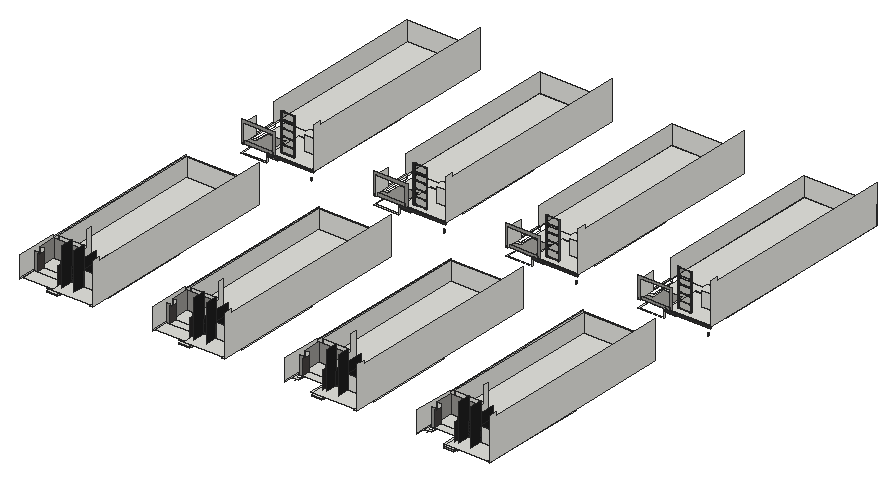
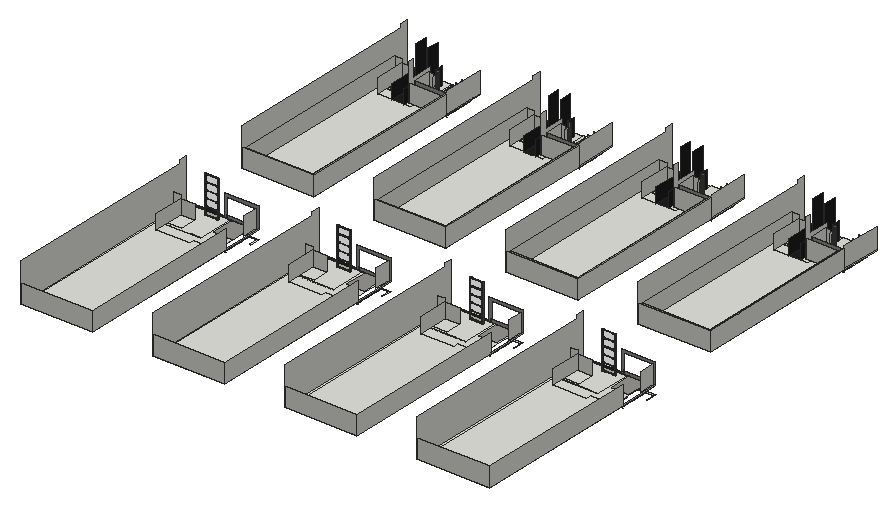
# SketchUp Ruby script. Lengths in inches.
U = 1.inch
M = Sketchup.active_model
def pt(a) = Geom::Point3d.new(a.map { |v| v * U })
def face(e, loops, mat)
  f = e.add_face(loops[0].map { |a| pt(a) })
  loops[1..].each { |l| e.add_face(l.map { |a| pt(a) }).erase! }
  f.material = f.back_material = mat if mat
  f
end
# faces: each face lists its corners as indices into pts; further lists are holes
def faces(e, pts, list, mat = nil) = list.each { |f| face(e, (f[0].is_a?(Array) ? f : [f]).map { |l| l.map { |i| pts[i] } }, mat) }
# xy, xz, yz: faces in a plane at the given z, y or x. An outline is a flat list of corners, or four numbers for a rectangle; further outlines are holes
def ring(l) = l.size == 4 ? [[l[0], l[1]], [l[2], l[1]], [l[2], l[3]], [l[0], l[3]]] : l.each_slice(2).to_a
def flat(e, list, mat, &to3) = list.each { |f| face(e, (f[0].is_a?(Array) ? f : [f]).map { |l| ring(l).map { |u, v| to3.(u, v) } }, mat) }
def xy(e, z, list, mat = nil) = flat(e, list, mat) { |x, y| [x, y, z] }
def xz(e, y, list, mat = nil) = flat(e, list, mat) { |x, z| [x, y, z] }
def yz(e, x, list, mat = nil) = flat(e, list, mat) { |y, z| [x, y, z] }
def lines(e, pts, list) = list.each { |a, b| e.add_line(pt(pts[a]), pt(pts[b])) }
# prism: a flat outline (further loops are holes) pulled along v
def prism(e, loops, v, mat = nil)
  f = face(e, loops, mat); d = Geom::Vector3d.new(v.map { |x| x * U })
  f.pushpull(f.normal.samedirection?(d) ? d.length : -d.length)
end
def box(e, o, s, mat = nil) = prism(e, [[o, [o[0] + s[0], o[1], o[2]], [o[0] + s[0], o[1] + s[1], o[2]], [o[0], o[1] + s[1], o[2]]]], [0, 0, s[2]], mat)
def at(x, y, z, deg = 0) = Geom::Transformation.translation(pt([x, y, z])) * Geom::Transformation.rotation(ORIGIN, Z_AXIS, deg.degrees)
def axes(o, x, y, z) = Geom::Transformation.new([*x, 0, *y, 0, *z, 0, *pt(o).to_a, 1])
def part(name) = M.definitions.add(name)
# library, detail: a bought-in or finely detailed component or shape, given as its bounding box
def library(name, o, s) = part(name).tap { |d| box(d.entities, o, s) }
def detail(e, o, s) = box(e.add_group.entities, o, s)
def put(e, d, t, mat = nil) = e.add_instance(d, t).tap { |i| i.material = mat if mat }
def group(e, t, mat = nil) = e.add_group.tap { |g| g.transformation = t; g.material = mat if mat }.entities
root = M.entities
M.materials.add("Aluminum_Polished").color = [83, 85, 85]
M.materials.add("Glass_Window_Neutral").color = [0, 0, 0]
M.materials["Glass_Window_Neutral"].alpha = 0.125
M.materials.add("[Color M07]").color = [58, 58, 58]
M.materials.add("[Color M08]").color = [30, 30, 30]
M.materials.add("[Field Square Tile]").color = [211, 167, 108]
M.materials.add("[Granite Dark Gray]").color = [38, 37, 37]
M.materials.add("[Granite Light Gray]").color = [149, 148, 144]
M.materials.add("[Granite Tile]1").color = [68, 65, 63]
c1 = part("Group\#7")
xy(c1.entities,0,[[6,0,4.45,0.2,3,0.8,1.76,1.76,0.8,3,0.2,4.45,0,6,0.2,7.55,0.8,9,1.76,10.24,3,11.2,4.45,11.8,6,12,7.55,11.8,9,11.2,10.24,10.24,11.2,9,11.8,7.55,12,6,11.8,4.45,11.2,3,10.24,1.76,9,0.8,7.55,0.2]])
xy(c1.entities,37,[[6,0,7.55,0.2,9,0.8,10.24,1.76,11.2,3,11.8,4.45,12,6,11.8,7.55,11.2,9,10.24,10.24,9,11.2,7.55,11.8,6,12,4.45,11.8,3,11.2,1.76,10.24,0.8,9,0.2,7.55,0,6,0.2,4.45,0.8,3,1.76,1.76,3,0.8,4.45,0.2]],"[Granite Tile]1")
p = [[4.45,0.2,0],[6,0,0],[6,0,37],[4.45,0.2,37],[7.55,0.2,0],[7.55,0.2,37],
  [3,0.8,0],[3,0.8,37],[9,0.8,0],[9,0.8,37],[1.76,1.76,0],[1.76,1.76,37],
  [10.24,1.76,0],[10.24,1.76,37],[0.8,3,0],[0.8,3,37],[11.2,3,0],[11.2,3,37],
  [0.2,4.45,0],[0.2,4.45,37],[11.8,4.45,0],[11.8,4.45,37],[0,6,0],[0,6,37],
  [12,6,0],[12,6,37],[0.2,7.55,0],[0.2,7.55,37],[11.8,7.55,0],[11.8,7.55,37],
  [0.8,9,0],[0.8,9,37],[11.2,9,0],[11.2,9,37],[1.76,10.24,0],[1.76,10.24,37],
  [10.24,10.24,0],[10.24,10.24,37],[3,11.2,0],[3,11.2,37],[9,11.2,0],[9,11.2,37],
  [4.45,11.8,0],[4.45,11.8,37],[7.55,11.8,0],[7.55,11.8,37],[6,12,0],[6,12,37]]
faces(c1.entities,p,[[0,1,2,3],[1,4,5,2],[6,0,3,7],[4,8,9,5],[10,6,7,11],[8,12,13,9],[14,10,11,15],[12,16,17,13],
  [18,14,15,19],[16,20,21,17],[22,18,19,23],[20,24,25,21],[26,22,23,27],[24,28,29,25],[30,26,27,31],[28,32,33,29],
  [34,30,31,35],[32,36,37,33],[38,34,35,39],[36,40,41,37],[42,38,39,43],[40,44,45,41],[46,42,43,47],[44,46,47,45]],"[Granite Tile]1")
c2 = part("Group\#54")
box(c2.entities,[0,0,0],[2,1,28])
c3 = part("Group\#56")
p = [[0.11,0.32,0.14],[0.11,0.69,0.14]]
lines(c3.entities,p,[[0,1]])
g1 = group(c3.entities,at(0.11,0,0))
prism(g1,[[[0,0.24,0],[0,0.32,0.14],[0,0.24,0.27],[0,0.08,0.27],[0,0,0.14],[0,0.08,0]]],[-0.11,0,0])
c4 = part("Ver Glass Railing")
g2 = group(c4.entities,at(0,0,0),"Aluminum_Polished")
box(g2,[0,0,0],[2,185,2])
g3 = group(c4.entities,at(0,0,2),"Aluminum_Polished")
p = [[1.41,1,0],[1.41,36.8,0],[1.41,184,0],[1.29,184,0],[1.29,1,0],[1.29,36.8,0],
  [1.41,184,28],[1.29,184,28],[1.41,148.2,28],[1.29,148.2,28],[1.41,1,28],[1.29,1,28],
  [1.29,111.4,28],[1.29,111.4,0],[1.41,111.4,0],[1.41,111.4,28],[1.29,110.4,0],[1.29,110.4,28],
  [1.41,110.4,28],[1.41,110.4,0],[1.29,74.6,28],[1.29,74.6,0],[1.41,74.6,0],[1.41,74.6,28],
  [1.29,73.6,0],[1.29,73.6,28],[1.41,73.6,28],[1.41,73.6,0],[1.29,148.2,0],[1.41,148.2,0],
  [1.29,147.2,0],[1.29,147.2,28],[1.41,147.2,28],[1.41,147.2,0],[1.29,37.8,28],[1.29,37.8,0],
  [1.41,37.8,0],[1.41,37.8,28],[1.29,36.8,28],[1.41,36.8,28]]
lines(g3,p,[[0,1],[2,3],[4,5],[6,7],[6,8],[7,9],[10,11],[2,6],[3,7],[0,4],[11,4],[10,0],
  [12,13],[14,15],[16,17],[18,19],[20,21],[22,23],[24,25],[26,27],[27,22],[24,21],[23,26],[20,25],
  [9,28],[29,8],[30,31],[32,33],[33,29],[30,28],[8,32],[9,31],[34,35],[36,37],[5,38],[39,1],
  [1,36],[5,35],[37,39],[14,33],[19,14],[22,19],[36,27],[13,30],[16,13],[21,16],[35,24],[15,18],
  [12,17],[29,2],[28,3],[18,23],[32,15],[17,20],[31,12],[26,37],[25,34],[34,38],[39,10],[38,11]])
g4 = group(g3,at(1.79,1,0))
box(g4,[-0.5,0,0],[0.125,183,28],"Glass_Window_Neutral")
g5 = group(g3,at(0,184,28))
box(g5,[0,-184,0],[2.5,185,1])
put(g3,c2,axes([2,185,28],[-1,0,0],[0,-1,0],[0,0,-1]))
put(g3,c2,axes([2,1,28],[-1,0,0],[0,-1,0],[0,0,-1]))
put(g3,c2,axes([2,111.4,28],[-1,0,0],[0,-1,0],[0,0,-1]))
put(g3,c2,axes([2,74.6,28],[-1,0,0],[0,-1,0],[0,0,-1]))
g6 = group(g3,at(2,148.2,28))
box(g6,[-2,-1,-28],[2,1,28])
put(g3,c2,axes([2,37.8,28],[-1,0,0],[0,-1,0],[0,0,-1]))
put(g3,c3,at(1.17,146.31,24.26))
put(g3,c3,axes([1.17,148.89,24.54],[1,0,0],[0,-1,0],[0,0,-1]))
put(g3,c3,axes([1.17,148.89,4.79],[1,0,0],[0,-1,0],[0,0,-1]))
put(g3,c3,at(1.17,146.31,4.51))
put(g3,c3,at(1.17,109.51,4.51))
put(g3,c3,axes([1.17,112.09,4.79],[1,0,0],[0,-1,0],[0,0,-1]))
put(g3,c3,axes([1.17,112.09,24.54],[1,0,0],[0,-1,0],[0,0,-1]))
put(g3,c3,at(1.17,109.51,24.26))
put(g3,c3,axes([1.17,75.29,24.54],[1,0,0],[0,-1,0],[0,0,-1]))
put(g3,c3,at(1.17,72.71,4.51))
put(g3,c3,axes([1.17,75.29,4.79],[1,0,0],[0,-1,0],[0,0,-1]))
put(g3,c3,at(1.17,72.71,24.26))
put(g3,c3,axes([1.17,38.49,24.54],[1,0,0],[0,-1,0],[0,0,-1]))
put(g3,c3,at(1.17,35.91,4.51))
put(g3,c3,axes([1.17,38.49,4.79],[1,0,0],[0,-1,0],[0,0,-1]))
put(g3,c3,at(1.17,35.91,24.26))
xy(root,72.4375,[[218.97,2293.1875,388.78,2293.1875,388.78,2300.94,225.79,2300.94,225.79,2358.81,218.97,2358.81],[1097.72,2293.1875,1267.53,2293.1875,1267.53,2300.94,1104.54,2300.94,1104.54,2358.81,1097.72,2358.81],[1976.47,2293.1875,2146.28,2293.1875,2146.28,2300.94,1983.29,2300.94,1983.29,2358.81,1976.47,2358.81],[2855.22,2293.1875,3025.03,2293.1875,3025.03,2300.94,2862.04,2300.94,2862.04,2358.81,2855.22,2358.81]])
xy(root,96.1875,[[402.97,706.62,460.85,1288.43],[1281.72,706.62,1339.6,1288.43],[2160.47,706.62,2218.35,1288.43],[3039.22,706.62,3097.1,1288.43],[402.97,2542.24,460.85,3124.06],
  [1281.72,2542.24,1339.6,3124.06],[2160.47,2542.24,2218.35,3124.06],[3039.22,2542.24,3097.1,3124.06]])
xy(root,96.29,[[488.9,633.06,669.8,1213.68],[1367.65,633.06,1548.55,1213.68],[2246.4,633.06,2427.3,1213.68],[3125.15,633.06,3306.05,1213.68],[488.9,2468.68,669.8,3049.31],
  [1367.65,2468.68,1548.55,3049.31],[2246.4,2468.68,2427.3,3049.31],[3125.15,2468.68,3306.05,3049.31]])
xy(root,107.07,[[279.88,619.06,385.01,1006.15],[1158.63,619.06,1263.76,1006.15],[2037.38,619.06,2142.51,1006.15],[2916.13,619.06,3021.26,1006.15],[279.88,2454.68,385.01,2841.77],
  [1158.63,2454.68,1263.76,2841.77],[2037.38,2454.68,2142.51,2841.77],[2916.13,2454.68,3021.26,2841.77]])
xy(root,110.32,[[395.95,458.5,463.7,706.62],[1274.7,458.5,1342.45,706.62],[2153.45,458.5,2221.2,706.62],[3032.2,458.5,3099.95,706.62],[395.95,2294.125,463.7,2542.24],
  [1274.7,2294.125,1342.45,2542.24],[2153.45,2294.125,2221.2,2542.24],[3032.2,2294.125,3099.95,2542.24]],"[Granite Light Gray]")
xy(root,116.94,[[481.29,561.06,678.9,571.64],[1360.04,561.06,1557.65,571.64],[2238.79,561.06,2436.4,571.64],[3117.54,561.06,3315.15,571.64],[481.29,2396.68,678.9,2407.27],
  [1360.04,2396.68,1557.65,2407.27],[2238.79,2396.68,2436.4,2407.27],[3117.54,2396.68,3315.15,2407.27]],"[Field Square Tile]")
xy(root,118.38,[[395.95,458.5,463.7,706.62],[1274.7,458.5,1342.45,706.62],[2153.45,458.5,2221.2,706.62],[3032.2,458.5,3099.95,706.62],[463.7,465.32,481.29,465.32,481.29,633.06,475.35,633.06,475.35,706.62,463.7,706.62],
  [1342.45,465.32,1360.04,465.32,1360.04,633.06,1354.1,633.06,1354.1,706.62,1342.45,706.62],[2221.2,465.32,2238.79,465.32,2238.79,633.06,2232.85,633.06,2232.85,706.62,2221.2,706.62],[3099.95,465.32,3117.54,465.32,3117.54,633.06,3111.6,633.06,3111.6,706.62,3099.95,706.62],[475.35,633.06,640.4,706.62],[640.4,633.06,678.9,706.62],
  [1354.1,633.06,1519.15,706.62],[1519.15,633.06,1557.65,706.62],[2232.85,633.06,2397.9,706.62],[2397.9,633.06,2436.4,706.62],[3111.6,633.06,3276.65,706.62],
  [3276.65,633.06,3315.15,706.62],[395.95,2294.125,463.7,2542.24],[463.7,2294.125,481.29,2300.94],[1274.7,2294.125,1342.45,2542.24],[1342.45,2294.125,1360.04,2300.94],
  [2153.45,2294.125,2221.2,2542.24],[2221.2,2294.125,2238.79,2300.94],[3032.2,2294.125,3099.95,2542.24],[3099.95,2294.125,3117.54,2300.94],[463.7,2300.94,481.29,2300.94,481.29,2468.68,475.35,2468.68,475.35,2542.24,463.7,2542.24],
  [1342.45,2300.94,1360.04,2300.94,1360.04,2468.68,1354.1,2468.68,1354.1,2542.24,1342.45,2542.24],[2221.2,2300.94,2238.79,2300.94,2238.79,2468.68,2232.85,2468.68,2232.85,2542.24,2221.2,2542.24],[3099.95,2300.94,3117.54,2300.94,3117.54,2468.68,3111.6,2468.68,3111.6,2542.24,3099.95,2542.24],[475.35,2468.68,640.4,2542.24],[640.4,2468.68,678.9,2542.24],
  [1354.1,2468.68,1519.15,2542.24],[1519.15,2468.68,1557.65,2542.24],[2232.85,2468.68,2397.9,2542.24],[2397.9,2468.68,2436.4,2542.24],[3111.6,2468.68,3276.65,2542.24],
  [3276.65,2468.68,3315.15,2542.24]])
xy(root,118.38,[[481.29,571.64,678.9,633.06],[1360.04,571.64,1557.65,633.06],[2238.79,571.64,2436.4,633.06],[3117.54,571.64,3315.15,633.06],[481.29,2294.125,678.9,2396.68],
  [1360.04,2294.125,1557.65,2396.68],[2238.79,2294.125,2436.4,2396.68],[3117.54,2294.125,3315.15,2396.68],[481.29,2407.27,678.9,2468.68],[1360.04,2407.27,1557.65,2468.68],
  [2238.79,2407.27,2436.4,2468.68],[3117.54,2407.27,3315.15,2468.68]],"[Granite Light Gray]")
xy(root,128.5,[[[678.9,458.5,698.16,458.5,698.16,1835.625,218.97,1835.625,218.97,523.18,262.66,523.18,262.66,619.06,388.78,619.06,388.78,463.25,399.95,463.25,399.95,706.62,678.9,706.62],[225.79,539.02,225.79,1828.81,678.9,1828.81,678.9,986.46,261.53,986.46,261.53,539.02]],[[1557.65,458.5,1576.91,458.5,1576.91,1835.625,1097.72,1835.625,1097.72,523.18,1141.41,523.18,1141.41,619.06,1267.53,619.06,1267.53,463.25,1278.7,463.25,1278.7,706.62,1557.65,706.62],[1104.54,539.02,1104.54,1828.81,1557.65,1828.81,1557.65,986.46,1140.28,986.46,1140.28,539.02]],[[2436.4,458.5,2455.66,458.5,2455.66,1835.625,1976.47,1835.625,1976.47,523.18,2020.16,523.18,2020.16,619.06,2146.28,619.06,2146.28,463.25,2157.45,463.25,2157.45,706.62,2436.4,706.62],[1983.29,539.02,1983.29,1828.81,2436.4,1828.81,2436.4,986.46,2019.03,986.46,2019.03,539.02]],[[3315.15,458.5,3334.41,458.5,3334.41,1835.625,2855.22,1835.625,2855.22,523.18,2898.91,523.18,2898.91,619.06,3025.03,619.06,3025.03,463.25,3036.2,463.25,3036.2,706.62,3315.15,706.62],[2862.04,539.02,2862.04,1828.81,3315.15,1828.81,3315.15,986.46,2897.78,986.46,2897.78,539.02]],[399.95,465.32,678.9,706.62],
  [1278.7,465.32,1557.65,706.62],[2157.45,465.32,2436.4,706.62],[3036.2,465.32,3315.15,706.62],[261.53,986.46,678.9,1006.15],[1140.28,986.46,1557.65,1006.15],
  [2019.03,986.46,2436.4,1006.15],[2897.78,986.46,3315.15,1006.15],[261.53,1006.15,678.9,1010.9],[1140.28,1006.15,1557.65,1010.9],[2019.03,1006.15,2436.4,1010.9],
  [2897.78,1006.15,3315.15,1010.9],[218.97,2294.125,225.79,2358.81],[[678.9,2294.125,698.16,2294.125,698.16,3671.25,218.97,3671.25,218.97,2358.81,262.66,2358.81,262.66,2454.68,388.78,2454.68,388.78,2298.875,399.95,2298.875,399.95,2542.24,678.9,2542.24],[225.79,2374.65,225.79,3664.43,678.9,3664.43,678.9,2822.08,261.53,2822.08,261.53,2374.65]],[388.78,2294.125,399.95,2298.875],[399.95,2294.125,427.1,2298.875],
  [427.1,2294.125,427.1,2298.875,399.95,2298.875,399.95,2300.94,678.9,2300.94,678.9,2294.125],[1097.72,2294.125,1104.54,2358.81],[[1557.65,2294.125,1576.91,2294.125,1576.91,3671.25,1097.72,3671.25,1097.72,2358.81,1141.41,2358.81,1141.41,2454.68,1267.53,2454.68,1267.53,2298.875,1278.7,2298.875,1278.7,2542.24,1557.65,2542.24],[1104.54,2374.65,1104.54,3664.43,1557.65,3664.43,1557.65,2822.08,1140.28,2822.08,1140.28,2374.65]],[1267.53,2294.125,1278.7,2298.875],[1278.7,2294.125,1305.85,2298.875],
  [1305.85,2294.125,1305.85,2298.875,1278.7,2298.875,1278.7,2300.94,1557.65,2300.94,1557.65,2294.125],[1976.47,2294.125,1983.29,2358.81],[[2436.4,2294.125,2455.66,2294.125,2455.66,3671.25,1976.47,3671.25,1976.47,2358.81,2020.16,2358.81,2020.16,2454.68,2146.28,2454.68,2146.28,2298.875,2157.45,2298.875,2157.45,2542.24,2436.4,2542.24],[1983.29,2374.65,1983.29,3664.43,2436.4,3664.43,2436.4,2822.08,2019.03,2822.08,2019.03,2374.65]],[2146.28,2294.125,2157.45,2298.875],[2157.45,2294.125,2184.6,2298.875],
  [2184.6,2294.125,2184.6,2298.875,2157.45,2298.875,2157.45,2300.94,2436.4,2300.94,2436.4,2294.125],[2855.22,2294.125,2862.04,2358.81],[[3315.15,2294.125,3334.41,2294.125,3334.41,3671.25,2855.22,3671.25,2855.22,2358.81,2898.91,2358.81,2898.91,2454.68,3025.03,2454.68,3025.03,2298.875,3036.2,2298.875,3036.2,2542.24,3315.15,2542.24],[2862.04,2374.65,2862.04,3664.43,3315.15,3664.43,3315.15,2822.08,2897.78,2822.08,2897.78,2374.65]],[3025.03,2294.125,3036.2,2298.875],[3036.2,2294.125,3063.35,2298.875],
  [3063.35,2294.125,3063.35,2298.875,3036.2,2298.875,3036.2,2300.94,3315.15,2300.94,3315.15,2294.125],[399.95,2300.94,678.9,2542.24],[1278.7,2300.94,1557.65,2542.24],[2157.45,2300.94,2436.4,2542.24],[3036.2,2300.94,3315.15,2542.24],
  [261.53,2822.08,678.9,2841.77],[1140.28,2822.08,1557.65,2841.77],[2019.03,2822.08,2436.4,2841.77],[2897.78,2822.08,3315.15,2841.77],[261.53,2841.77,678.9,2846.52],
  [1140.28,2841.77,1557.65,2846.52],[2019.03,2841.77,2436.4,2846.52],[2897.78,2841.77,3315.15,2846.52]])
xy(root,128.5,[[228.78,2294.125,228.78,2358.81,262.66,2358.81,262.66,2454.68,388.78,2454.68,388.78,2298.875,232.96,2298.875,232.96,2294.125],[1107.53,2294.125,1107.53,2358.81,1141.41,2358.81,1141.41,2454.68,1267.53,2454.68,1267.53,2298.875,1111.71,2298.875,1111.71,2294.125],[1986.28,2294.125,1986.28,2358.81,2020.16,2358.81,2020.16,2454.68,2146.28,2454.68,2146.28,2298.875,1990.46,2298.875,1990.46,2294.125],[2865.03,2294.125,2865.03,2358.81,2898.91,2358.81,2898.91,2454.68,3025.03,2454.68,3025.03,2298.875,2869.21,2298.875,2869.21,2294.125]],"[Granite Light Gray]")
xy(root,134.5,[[232.96,468.31,427.1,561.05],[1111.71,468.31,1305.85,561.05],[252.78,561.05,406.85,611.02],[1131.53,561.05,1285.6,611.02],[2010.28,561.05,2164.35,611.02],
  [2889.03,561.05,3043.1,611.02],[629.77,589.83,676.54,589.83,676.54,1825.82,228.78,1825.82,228.78,762.17,406.85,762.17,406.85,792.52,629.77,792.52],[406.85,589.83,406.85,611.02,433.97,611.02,433.97,697.21,444.78,697.21,444.78,589.83],[444.78,589.83,453.7,697.21],[534.46,589.83,629.77,697.21],
  [1508.52,589.83,1555.29,589.83,1555.29,1825.82,1107.53,1825.82,1107.53,762.17,1285.6,762.17,1285.6,792.52,1508.52,792.52],[1285.6,589.83,1285.6,611.02,1312.72,611.02,1312.72,697.21,1323.53,697.21,1323.53,589.83],[1323.53,589.83,1332.45,697.21],[1413.21,589.83,1508.52,697.21],[2387.27,589.83,2434.04,589.83,2434.04,1825.82,1986.28,1825.82,1986.28,762.17,2164.35,762.17,2164.35,792.52,2387.27,792.52],
  [2164.35,589.83,2164.35,611.02,2191.47,611.02,2191.47,697.21,2202.28,697.21,2202.28,589.83],[2202.28,589.83,2211.2,697.21],[2291.96,589.83,2387.27,697.21],[3266.02,589.83,3312.79,589.83,3312.79,1825.82,2865.03,1825.82,2865.03,762.17,3043.1,762.17,3043.1,792.52,3266.02,792.52],[3043.1,589.83,3043.1,611.02,3070.22,611.02,3070.22,697.21,3081.03,697.21,3081.03,589.83],
  [3081.03,589.83,3089.95,697.21],[3170.71,589.83,3266.02,697.21],[228.78,611.02,406.85,727.2],[406.85,611.02,433.97,697.21],[1107.53,611.02,1285.6,727.2],
  [1285.6,611.02,1312.72,697.21],[1986.28,611.02,2164.35,727.2],[2164.35,611.02,2191.47,697.21],[2865.03,611.02,3043.1,727.2],[3043.1,611.02,3070.22,697.21],
  [406.85,697.21,433.97,727.2],[433.97,697.21,433.97,727.2,406.85,727.2,406.85,762.17,444.78,762.17,444.78,697.21],[444.78,697.21,453.7,697.21,453.7,792.52,406.85,792.52,406.85,762.17,444.78,762.17],[1285.6,697.21,1312.72,727.2],[1312.72,697.21,1312.72,727.2,1285.6,727.2,1285.6,762.17,1323.53,762.17,1323.53,697.21],
  [1323.53,697.21,1332.45,697.21,1332.45,792.52,1285.6,792.52,1285.6,762.17,1323.53,762.17],[2164.35,697.21,2191.47,727.2],[2191.47,697.21,2191.47,727.2,2164.35,727.2,2164.35,762.17,2202.28,762.17,2202.28,697.21],[2202.28,697.21,2211.2,697.21,2211.2,792.52,2164.35,792.52,2164.35,762.17,2202.28,762.17],[3043.1,697.21,3070.22,727.2],
  [3070.22,697.21,3070.22,727.2,3043.1,727.2,3043.1,762.17,3081.03,762.17,3081.03,697.21],[3081.03,697.21,3089.95,697.21,3089.95,792.52,3043.1,792.52,3043.1,762.17,3081.03,762.17],[629.77,2425.46,676.54,2425.46,676.54,3661.44,228.78,3661.44,228.78,2597.8,406.85,2597.8,406.85,2628.15,629.77,2628.15],[534.46,2425.46,629.77,2532.83],[1508.52,2425.46,1555.29,2425.46,1555.29,3661.44,1107.53,3661.44,1107.53,2597.8,1285.6,2597.8,1285.6,2628.15,1508.52,2628.15],
  [1413.21,2425.46,1508.52,2532.83],[2387.27,2425.46,2434.04,2425.46,2434.04,3661.44,1986.28,3661.44,1986.28,2597.8,2164.35,2597.8,2164.35,2628.15,2387.27,2628.15],[2291.96,2425.46,2387.27,2532.83],[3266.02,2425.46,3312.79,2425.46,3312.79,3661.44,2865.03,3661.44,2865.03,2597.8,3043.1,2597.8,3043.1,2628.15,3266.02,2628.15],[3170.71,2425.46,3266.02,2532.83]])
xy(root,134.5,[[453.7,589.83,534.46,792.52],[1332.45,589.83,1413.21,792.52],[2211.2,589.83,2291.96,792.52],[3089.95,589.83,3170.71,792.52]],"[Color M08]")
xz(root,561.05,[[232.96,134.5,252.78,251.5],[406.85,134.5,427.1,251.5],[1111.71,134.5,1131.53,251.5],[1285.6,134.5,1305.85,251.5],[1990.46,134.5,2010.28,251.5],
  [2164.35,134.5,2184.6,251.5],[2869.21,134.5,2889.03,251.5],[3043.1,134.5,3063.35,251.5]],"[Granite Light Gray]")
xz(root,561.06,[[481.29,116.94,678.9,118.38],[1360.04,116.94,1557.65,118.38],[2238.79,116.94,2436.4,118.38],[3117.54,116.94,3315.15,118.38]],"[Field Square Tile]")
xz(root,571.64,[[481.29,116.94,678.9,118.38],[1360.04,116.94,1557.65,118.38],[2238.79,116.94,2436.4,118.38],[3117.54,116.94,3315.15,118.38]],"[Field Square Tile]")
xz(root,589.83,[[406.85,134.5,444.78,231],[444.78,134.5,453.7,231],[534.46,134.5,629.77,231],[629.77,134.5,676.54,254.5],[1285.6,134.5,1323.53,231],
  [1323.53,134.5,1332.45,231],[1413.21,134.5,1508.52,231],[1508.52,134.5,1555.29,254.5],[2164.35,134.5,2202.28,231],[2202.28,134.5,2211.2,231],
  [2291.96,134.5,2387.27,231],[2387.27,134.5,2434.04,254.5],[3043.1,134.5,3081.03,231],[3081.03,134.5,3089.95,231],[3170.71,134.5,3266.02,231],
  [3266.02,134.5,3312.79,254.5]])
xz(root,611.02,[[228.78,134.5,252.78,254.5],[406.85,134.5,433.97,254.5],[1107.53,134.5,1131.53,254.5],[1285.6,134.5,1312.72,254.5],[1986.28,134.5,2010.28,254.5],
  [2164.35,134.5,2191.47,254.5],[2865.03,134.5,2889.03,254.5],[3043.1,134.5,3070.22,254.5]])
xz(root,706.62,[[395.95,110.32,399.95,118.38],[399.95,110.32,463.7,118.38],[1274.7,110.32,1278.7,118.38],[1278.7,110.32,1342.45,118.38],[2153.45,110.32,2157.45,118.38],
  [2157.45,110.32,2221.2,118.38],[3032.2,110.32,3036.2,118.38],[3036.2,110.32,3099.95,118.38],[399.95,118.38,463.7,128.5],[463.7,118.38,475.35,128.5],
  [475.35,118.38,640.4,128.5],[640.4,118.38,678.9,128.5],[1278.7,118.38,1342.45,128.5],[1342.45,118.38,1354.1,128.5],[1354.1,118.38,1519.15,128.5],
  [1519.15,118.38,1557.65,128.5],[2157.45,118.38,2221.2,128.5],[2221.2,118.38,2232.85,128.5],[2232.85,118.38,2397.9,128.5],[2397.9,118.38,2436.4,128.5],
  [3036.2,118.38,3099.95,128.5],[3099.95,118.38,3111.6,128.5],[3111.6,118.38,3276.65,128.5],[3276.65,118.38,3315.15,128.5]])
xz(root,727.2,[[228.78,134.5,433.97,254.5],[1107.53,134.5,1312.72,254.5],[1986.28,134.5,2191.47,254.5],[2865.03,134.5,3070.22,254.5]],"[Granite Light Gray]")
xz(root,762.17,[[228.78,134.5,444.78,254.5],[1107.53,134.5,1323.53,254.5],[1986.28,134.5,2202.28,254.5],[2865.03,134.5,3081.03,254.5]])
xz(root,1825.82,[[228.78,134.5,676.54,254.5],[1107.53,134.5,1555.29,254.5],[1986.28,134.5,2434.04,254.5],[2865.03,134.5,3312.79,254.5]])
xz(root,1835.625,[[218.97,128.5,698.16,254.5],[1097.72,128.5,1576.91,254.5],[1976.47,128.5,2455.66,254.5],[2855.22,128.5,3334.41,254.5]])
xz(root,2294.125,[[388.78,118.38,698.16,128.5],[1267.53,118.38,1576.91,128.5],[2146.28,118.38,2455.66,128.5],[3025.03,118.38,3334.41,128.5],[442.35,128.5,698.16,134.5],
  [1321.1,128.5,1576.91,134.5],[2199.85,128.5,2455.66,134.5],[3078.6,128.5,3334.41,134.5]],"[Color M07]")
xz(root,2294.125,[[218.97,128.5,232.96,128.5,232.96,251.5,427.1,251.5,427.1,128.5,442.35,128.5,442.35,270.8125,218.97,270.8125],[1097.72,128.5,1111.71,128.5,1111.71,251.5,1305.85,251.5,1305.85,128.5,1321.1,128.5,1321.1,270.8125,1097.72,270.8125],[1976.47,128.5,1990.46,128.5,1990.46,251.5,2184.6,251.5,2184.6,128.5,2199.85,128.5,2199.85,270.8125,1976.47,270.8125],[2855.22,128.5,2869.21,128.5,2869.21,251.5,3063.35,251.5,3063.35,128.5,3078.6,128.5,3078.6,270.8125,2855.22,270.8125]],"[Granite Light Gray]")
xz(root,2298.875,[[232.96,128.5,427.1,147.6875],[1111.71,128.5,1305.85,147.6875],[1990.46,128.5,2184.6,147.6875],[2869.21,128.5,3063.35,147.6875]],"[Granite Light Gray]")
xz(root,2396.68,[[481.29,116.94,678.9,118.38],[1360.04,116.94,1557.65,118.38],[2238.79,116.94,2436.4,118.38],[3117.54,116.94,3315.15,118.38]],"[Field Square Tile]")
xz(root,2407.27,[[481.29,116.94,678.9,118.38],[1360.04,116.94,1557.65,118.38],[2238.79,116.94,2436.4,118.38],[3117.54,116.94,3315.15,118.38]],"[Field Square Tile]")
xz(root,2425.46,[[534.46,134.5,629.77,231],[629.77,134.5,676.54,254.5],[1413.21,134.5,1508.52,231],[1508.52,134.5,1555.29,254.5],[2291.96,134.5,2387.27,231],
  [2387.27,134.5,2434.04,254.5],[3170.71,134.5,3266.02,231],[3266.02,134.5,3312.79,254.5]])
xz(root,2542.24,[[395.95,110.32,399.95,118.38],[399.95,110.32,463.7,118.38],[1274.7,110.32,1278.7,118.38],[1278.7,110.32,1342.45,118.38],[2153.45,110.32,2157.45,118.38],
  [2157.45,110.32,2221.2,118.38],[3032.2,110.32,3036.2,118.38],[3036.2,110.32,3099.95,118.38],[399.95,118.38,463.7,128.5],[463.7,118.38,475.35,128.5],
  [475.35,118.38,640.4,128.5],[640.4,118.38,678.9,128.5],[1278.7,118.38,1342.45,128.5],[1342.45,118.38,1354.1,128.5],[1354.1,118.38,1519.15,128.5],
  [1519.15,118.38,1557.65,128.5],[2157.45,118.38,2221.2,128.5],[2221.2,118.38,2232.85,128.5],[2232.85,118.38,2397.9,128.5],[2397.9,118.38,2436.4,128.5],
  [3036.2,118.38,3099.95,128.5],[3099.95,118.38,3111.6,128.5],[3111.6,118.38,3276.65,128.5],[3276.65,118.38,3315.15,128.5]])
xz(root,3671.25,[[218.97,128.5,698.16,254.5],[1097.72,128.5,1576.91,254.5],[1976.47,128.5,2455.66,254.5],[2855.22,128.5,3334.41,254.5]])
yz(root,218.97,[[458.5,128.5,727.2,134.5],[727.2,128.5,1835.625,254.5],[2294.125,128.5,2562.82,134.5],[2562.82,128.5,3671.25,254.5],[458.5,134.5,458.5,270.8125,727.2,270.8125,727.2,260.5,1835.625,260.5,1835.625,254.5,727.2,254.5,727.2,134.5]])
yz(root,228.78,[[762.17,134.5,1825.82,254.5]])
yz(root,228.78,[[611.02,134.5,727.2,254.5]],"[Granite Light Gray]")
yz(root,232.96,[[2294.125,128.5,2298.875,128.5,2298.875,147.6875,2303.93,147.6875,2303.93,134.5,2396.68,134.5,2396.68,251.5,2294.125,251.5]])
yz(root,252.78,[[561.05,134.5,611.02,134.5,611.02,230.89,566.68,230.89,566.68,241.52,561.05,241.52]],"[Granite Tile]1")
yz(root,388.78,[[2294.125,72.4375,2300.94,128.5]])
yz(root,406.85,[[589.83,134.5,611.02,230.89]])
yz(root,406.85,[[561.05,134.5,561.05,240.93,564.15,241.17,564.19,241.17,564.18,241.17,565.74,241.29,565.74,240.89,566.68,240.89,566.68,230.89,589.83,230.89,589.83,134.5]],"[Granite Tile]1")
yz(root,427.1,[[2294.125,128.5,2298.875,147.6875]])
yz(root,427.1,[[511.08,134.5,561.05,251.5]],"[Granite Dark Gray]")
yz(root,433.97,[[611.02,134.5,727.2,254.5]])
yz(root,444.78,[[589.83,134.5,762.17,134.5,762.17,380.5,727.2,380.5,727.2,270.8125,589.83,270.8125]])
yz(root,453.7,[[511.08,134.5,589.83,380.5],[589.83,134.5,792.52,231]],"[Color M08]")
yz(root,463.7,[[465.32,110.32,706.62,118.38],[2294.125,110.32,2300.94,118.38],[2300.94,110.32,2542.24,118.38]])
yz(root,481.29,[[561.06,116.94,571.64,118.38],[2396.68,116.94,2407.27,118.38]],"[Field Square Tile]")
yz(root,534.46,[[511.08,134.5,589.83,380.5],[589.83,134.5,792.52,231]],"[Color M08]")
yz(root,629.77,[[589.83,134.5,792.52,231],[2425.46,134.5,2628.15,231]])
yz(root,676.54,[[589.83,134.5,1825.82,254.5]])
yz(root,698.16,[[458.5,128.5,1835.625,128.5,1835.625,380.5,511.08,380.5,511.08,403.8125,458.5,403.8125],[2294.125,128.5,3671.25,128.5,3671.25,380.5,2346.71,380.5,2346.71,403.8125,2294.125,403.8125]])
yz(root,1097.72,[[458.5,128.5,727.2,134.5],[727.2,128.5,1835.625,254.5],[2294.125,128.5,2562.82,134.5],[2562.82,128.5,3671.25,254.5],[458.5,134.5,458.5,270.8125,727.2,270.8125,727.2,260.5,1835.625,260.5,1835.625,254.5,727.2,254.5,727.2,134.5]])
yz(root,1107.53,[[762.17,134.5,1825.82,254.5]])
yz(root,1107.53,[[611.02,134.5,727.2,254.5]],"[Granite Light Gray]")
yz(root,1111.71,[[2294.125,128.5,2298.875,128.5,2298.875,147.6875,2303.93,147.6875,2303.93,134.5,2396.68,134.5,2396.68,251.5,2294.125,251.5]])
yz(root,1131.53,[[561.05,134.5,611.02,134.5,611.02,230.89,566.68,230.89,566.68,241.52,561.05,241.52]],"[Granite Tile]1")
yz(root,1267.53,[[2294.125,72.4375,2300.94,128.5]])
yz(root,1285.6,[[589.83,134.5,611.02,230.89]])
yz(root,1285.6,[[561.05,134.5,561.05,240.93,564.15,241.17,564.19,241.17,564.18,241.17,565.74,241.29,565.74,240.89,566.68,240.89,566.68,230.89,589.83,230.89,589.83,134.5]],"[Granite Tile]1")
yz(root,1305.85,[[2294.125,128.5,2298.875,147.6875]])
yz(root,1305.85,[[511.08,134.5,561.05,251.5]],"[Granite Dark Gray]")
yz(root,1312.72,[[611.02,134.5,727.2,254.5]])
yz(root,1323.53,[[589.83,134.5,762.17,134.5,762.17,380.5,727.2,380.5,727.2,270.8125,589.83,270.8125]])
yz(root,1332.45,[[511.08,134.5,589.83,380.5],[589.83,134.5,792.52,231]],"[Color M08]")
yz(root,1342.45,[[465.32,110.32,706.62,118.38],[2294.125,110.32,2300.94,118.38],[2300.94,110.32,2542.24,118.38]])
yz(root,1360.04,[[561.06,116.94,571.64,118.38],[2396.68,116.94,2407.27,118.38]],"[Field Square Tile]")
yz(root,1413.21,[[511.08,134.5,589.83,380.5],[589.83,134.5,792.52,231]],"[Color M08]")
yz(root,1508.52,[[589.83,134.5,792.52,231],[2425.46,134.5,2628.15,231]])
yz(root,1555.29,[[589.83,134.5,1825.82,254.5]])
yz(root,1576.91,[[458.5,128.5,1835.625,128.5,1835.625,380.5,511.08,380.5,511.08,403.8125,458.5,403.8125],[2294.125,128.5,3671.25,128.5,3671.25,380.5,2346.71,380.5,2346.71,403.8125,2294.125,403.8125]])
yz(root,1976.47,[[458.5,128.5,727.2,134.5],[727.2,128.5,1835.625,254.5],[2294.125,128.5,2562.82,134.5],[2562.82,128.5,3671.25,254.5],[458.5,134.5,458.5,270.8125,727.2,270.8125,727.2,260.5,1835.625,260.5,1835.625,254.5,727.2,254.5,727.2,134.5]])
yz(root,1986.28,[[762.17,134.5,1825.82,254.5]])
yz(root,1986.28,[[611.02,134.5,727.2,254.5]],"[Granite Light Gray]")
yz(root,1990.46,[[2294.125,128.5,2298.875,128.5,2298.875,147.6875,2303.93,147.6875,2303.93,134.5,2396.68,134.5,2396.68,251.5,2294.125,251.5]])
yz(root,2010.28,[[561.05,134.5,611.02,134.5,611.02,230.89,566.68,230.89,566.68,241.52,561.05,241.52]],"[Granite Tile]1")
yz(root,2146.28,[[2294.125,72.4375,2300.94,128.5]])
yz(root,2164.35,[[589.83,134.5,611.02,230.89]])
yz(root,2164.35,[[561.05,134.5,561.05,240.93,564.15,241.17,564.19,241.17,564.18,241.17,565.74,241.29,565.74,240.89,566.68,240.89,566.68,230.89,589.83,230.89,589.83,134.5]],"[Granite Tile]1")
yz(root,2184.6,[[2294.125,128.5,2298.875,147.6875]])
yz(root,2184.6,[[511.08,134.5,561.05,251.5]],"[Granite Dark Gray]")
yz(root,2191.47,[[611.02,134.5,727.2,254.5]])
yz(root,2202.28,[[589.83,134.5,762.17,134.5,762.17,380.5,727.2,380.5,727.2,270.8125,589.83,270.8125]])
yz(root,2211.2,[[511.08,134.5,589.83,380.5],[589.83,134.5,792.52,231]],"[Color M08]")
yz(root,2221.2,[[465.32,110.32,706.62,118.38],[2294.125,110.32,2300.94,118.38],[2300.94,110.32,2542.24,118.38]])
yz(root,2238.79,[[561.06,116.94,571.64,118.38],[2396.68,116.94,2407.27,118.38]],"[Field Square Tile]")
yz(root,2291.96,[[511.08,134.5,589.83,380.5],[589.83,134.5,792.52,231]],"[Color M08]")
yz(root,2387.27,[[589.83,134.5,792.52,231],[2425.46,134.5,2628.15,231]])
yz(root,2434.04,[[589.83,134.5,1825.82,254.5]])
yz(root,2455.66,[[458.5,128.5,1835.625,128.5,1835.625,380.5,511.08,380.5,511.08,403.8125,458.5,403.8125],[2294.125,128.5,3671.25,128.5,3671.25,380.5,2346.71,380.5,2346.71,403.8125,2294.125,403.8125]])
yz(root,2855.22,[[458.5,128.5,727.2,134.5],[727.2,128.5,1835.625,254.5],[2294.125,128.5,2562.82,134.5],[2562.82,128.5,3671.25,254.5],[458.5,134.5,458.5,270.8125,727.2,270.8125,727.2,260.5,1835.625,260.5,1835.625,254.5,727.2,254.5,727.2,134.5]])
yz(root,2865.03,[[762.17,134.5,1825.82,254.5]])
yz(root,2865.03,[[611.02,134.5,727.2,254.5]],"[Granite Light Gray]")
yz(root,2869.21,[[2294.125,128.5,2298.875,128.5,2298.875,147.6875,2303.93,147.6875,2303.93,134.5,2396.68,134.5,2396.68,251.5,2294.125,251.5]])
yz(root,2889.03,[[561.05,134.5,611.02,134.5,611.02,230.89,566.68,230.89,566.68,241.52,561.05,241.52]],"[Granite Tile]1")
yz(root,3025.03,[[2294.125,72.4375,2300.94,128.5]])
yz(root,3043.1,[[589.83,134.5,611.02,230.89]])
yz(root,3043.1,[[561.05,134.5,561.05,240.93,564.15,241.17,564.19,241.17,564.18,241.17,565.74,241.29,565.74,240.89,566.68,240.89,566.68,230.89,589.83,230.89,589.83,134.5]],"[Granite Tile]1")
yz(root,3063.35,[[2294.125,128.5,2298.875,147.6875]])
yz(root,3063.35,[[511.08,134.5,561.05,251.5]],"[Granite Dark Gray]")
yz(root,3070.22,[[611.02,134.5,727.2,254.5]])
yz(root,3081.03,[[589.83,134.5,762.17,134.5,762.17,380.5,727.2,380.5,727.2,270.8125,589.83,270.8125]])
yz(root,3089.95,[[511.08,134.5,589.83,380.5],[589.83,134.5,792.52,231]],"[Color M08]")
yz(root,3099.95,[[465.32,110.32,706.62,118.38],[2294.125,110.32,2300.94,118.38],[2300.94,110.32,2542.24,118.38]])
yz(root,3117.54,[[561.06,116.94,571.64,118.38],[2396.68,116.94,2407.27,118.38]],"[Field Square Tile]")
yz(root,3170.71,[[511.08,134.5,589.83,380.5],[589.83,134.5,792.52,231]],"[Color M08]")
yz(root,3266.02,[[589.83,134.5,792.52,231],[2425.46,134.5,2628.15,231]])
yz(root,3312.79,[[589.83,134.5,1825.82,254.5]])
yz(root,3334.41,[[458.5,128.5,1835.625,128.5,1835.625,380.5,511.08,380.5,511.08,403.8125,458.5,403.8125],[2294.125,128.5,3671.25,128.5,3671.25,380.5,2346.71,380.5,2346.71,403.8125,2294.125,403.8125]])
p = [[1976.68,1835.625,129.625],[1976.47,1835.625,128.5],[1976.47,727.2,134.5],[1986.28,727.2,134.5],[1986.28,727.2,113.375],[1976.47,727.2,113.375],
  [1986.28,523.18,113.375],[2436.4,571.64,118.38],[2444.29,571.64,118.38],[2855.43,1835.625,129.625],[2855.22,1835.625,128.5],[2855.22,727.2,134.5],
  [2865.03,727.2,134.5],[2865.03,727.2,113.375],[2865.03,523.18,113.375],[2855.22,727.2,113.375],[3315.15,571.64,118.38],[3323.04,571.64,118.38],
  [219.18,1835.625,129.625],[218.97,1835.625,128.5],[218.97,727.2,134.5],[228.78,727.2,134.5],[228.78,727.2,113.375],[228.78,523.18,113.375],
  [218.97,727.2,113.375],[1097.93,1835.625,129.625],[1097.72,1835.625,128.5],[1107.53,727.2,113.375],[1107.53,523.18,113.375],[1097.72,727.2,113.375],
  [1097.72,727.2,134.5],[1107.53,727.2,134.5],[678.9,571.64,118.38],[686.79,571.64,118.38],[1557.65,571.64,118.38],[1565.54,571.64,118.38],
  [2436.4,2300.94,118.38],[2436.4,2300.94,128.5],[1976.68,3671.25,129.625],[1976.47,3671.25,128.5],[1976.47,2562.82,134.5],[1986.28,2562.82,134.5],
  [1986.28,2562.82,113.375],[1986.28,2358.81,113.375],[1976.47,2562.82,113.375],[2435.48,2346.71,134.5],[2443.85,2346.71,134.5],[2855.43,3671.25,129.625],
  [2855.22,3671.25,128.5],[2865.03,2562.82,113.375],[2865.03,2358.81,113.375],[2855.22,2562.82,113.375],[2855.22,2562.82,134.5],[2865.03,2562.82,134.5],
  [3315.15,2300.94,118.38],[3315.15,2300.94,128.5],[2436.4,2407.27,118.38],[2444.29,2407.27,118.38],[678.9,2300.94,118.38],[678.9,2300.94,128.5],
  [219.18,3671.25,129.625],[218.97,3671.25,128.5],[3315.15,2407.27,118.38],[3323.04,2407.27,118.38],[677.98,2346.71,134.5],[686.35,2346.71,134.5],
  [228.78,2562.82,134.5],[228.78,2562.82,113.375],[1097.93,3671.25,129.625],[1097.72,3671.25,128.5],[1097.72,2562.82,134.5],[1107.53,2562.82,134.5],
  [1107.53,2562.82,113.375],[1107.53,2358.81,113.375],[1097.72,2562.82,113.375],[1557.65,2300.94,118.38],[1557.65,2300.94,128.5],[678.9,2407.27,118.38],
  [686.79,2407.27,118.38],[3314.23,2346.71,134.5],[3322.6,2346.71,134.5],[228.78,2358.81,113.375],[218.97,2562.82,134.5],[218.97,2562.82,113.375],
  [1556.73,2346.71,134.5],[1565.1,2346.71,134.5],[1557.65,2407.27,118.38],[1565.54,2407.27,118.38]]
lines(root,p,[[0,1],[2,3],[3,4],[5,4],[4,6],[7,8],[9,10],[11,12],[13,14],[15,13],[12,13],[16,17],
  [18,19],[20,21],[22,23],[24,22],[21,22],[25,26],[27,28],[29,27],[30,31],[32,33],[34,35],[31,27],
  [36,37],[38,39],[40,41],[42,43],[44,42],[45,46],[41,42],[47,48],[49,50],[51,49],[52,53],[54,55],
  [56,57],[58,59],[60,61],[62,63],[64,65],[66,67],[68,69],[70,71],[72,73],[74,72],[75,76],[77,78],
  [79,80],[53,49],[67,81],[82,66],[83,67],[84,85],[71,72],[86,87]])
put(root,c1,axes([2443.36,2289.09,72.9375],[0.42,0,0],[0,0.42,0],[0,0,0.42]))
put(root,c1,axes([3322.11,2289.09,72.9375],[0.42,0,0],[0,0.42,0],[0,0,0.42]))
put(root,c1,axes([685.86,2289.09,72.9375],[0.42,0,0],[0,0.42,0],[0,0,0.42]))
put(root,c1,axes([1564.61,2289.09,72.9375],[0.42,0,0],[0,0.42,0],[0,0,0.42]))
put(root,c4,axes([2201.18,2340.63,132.28],[0,1.33,0],[0,0,1.33],[2.92826,0,0]),"[Granite Dark Gray]")
put(root,c4,axes([443.68,2340.63,132.28],[0,1.33,0],[0,0,1.33],[2.92826,0,0]),"[Granite Dark Gray]")
put(root,c4,axes([1322.43,2340.63,132.28],[0,1.33,0],[0,0,1.33],[2.92826,0,0]),"[Granite Dark Gray]")
put(root,c4,axes([3079.93,2340.63,132.28],[0,1.33,0],[0,0,1.33],[2.92826,0,0]),"[Granite Dark Gray]")
